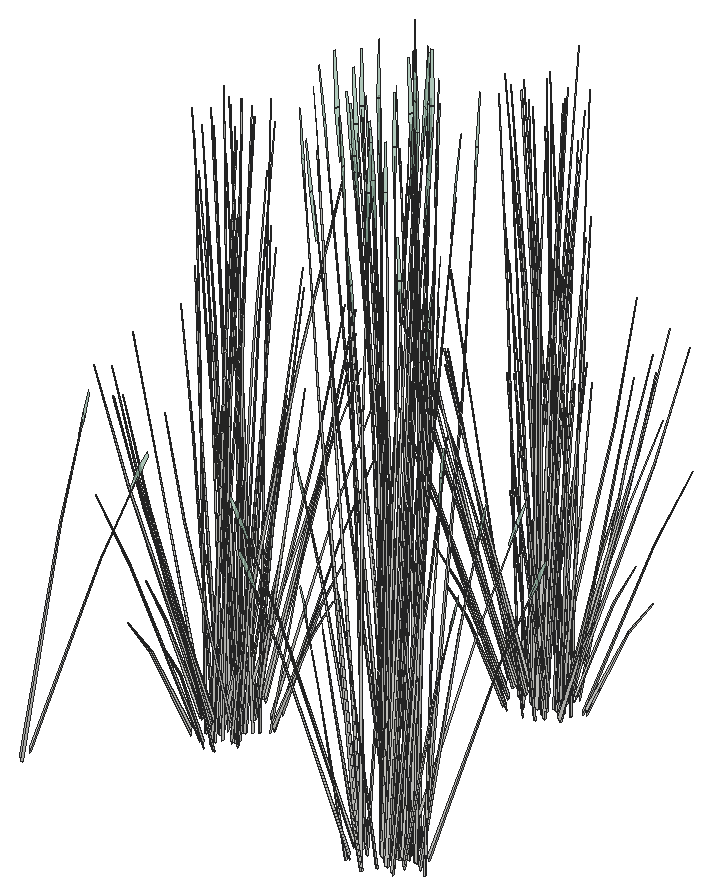
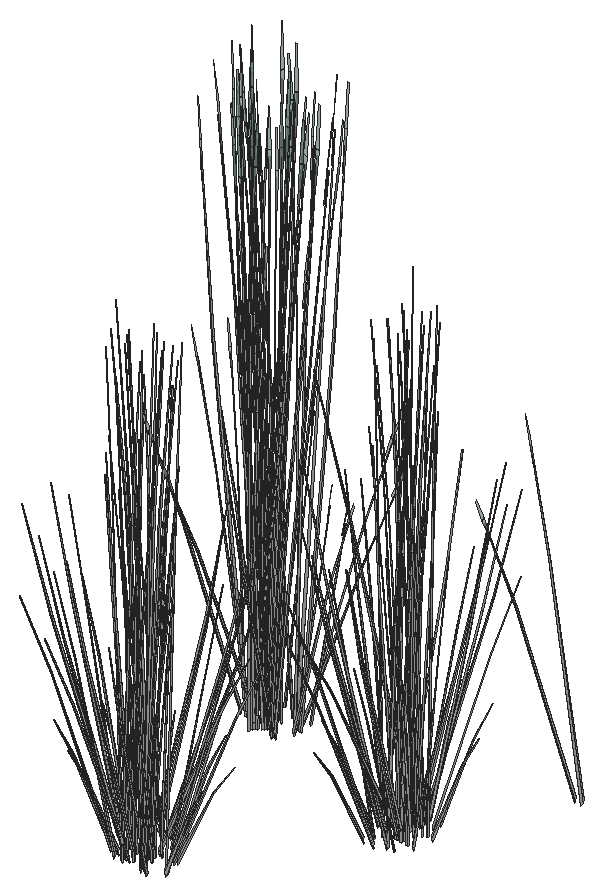
# SketchUp Ruby script. Lengths in inches.
U = 1.inch
M = Sketchup.active_model
def pt(a) = Geom::Point3d.new(a.map { |v| v * U })
def face(e, loops, mat)
  f = e.add_face(loops[0].map { |a| pt(a) })
  loops[1..].each { |l| e.add_face(l.map { |a| pt(a) }).erase! }
  f.material = f.back_material = mat if mat
  f
end
# faces: each face lists its corners as indices into pts; further lists are holes
def faces(e, pts, list, mat = nil) = list.each { |f| face(e, (f[0].is_a?(Array) ? f : [f]).map { |l| l.map { |i| pts[i] } }, mat) }
# xy, xz, yz: faces in a plane at the given z, y or x. An outline is a flat list of corners, or four numbers for a rectangle; further outlines are holes
def ring(l) = l.size == 4 ? [[l[0], l[1]], [l[2], l[1]], [l[2], l[3]], [l[0], l[3]]] : l.each_slice(2).to_a
def flat(e, list, mat, &to3) = list.each { |f| face(e, (f[0].is_a?(Array) ? f : [f]).map { |l| ring(l).map { |u, v| to3.(u, v) } }, mat) }
def xy(e, z, list, mat = nil) = flat(e, list, mat) { |x, y| [x, y, z] }
def xz(e, y, list, mat = nil) = flat(e, list, mat) { |x, z| [x, y, z] }
def yz(e, x, list, mat = nil) = flat(e, list, mat) { |y, z| [x, y, z] }
def lines(e, pts, list) = list.each { |a, b| e.add_line(pt(pts[a]), pt(pts[b])) }
# prism: a flat outline (further loops are holes) pulled along v
def prism(e, loops, v, mat = nil)
  f = face(e, loops, mat); d = Geom::Vector3d.new(v.map { |x| x * U })
  f.pushpull(f.normal.samedirection?(d) ? d.length : -d.length)
end
def box(e, o, s, mat = nil) = prism(e, [[o, [o[0] + s[0], o[1], o[2]], [o[0] + s[0], o[1] + s[1], o[2]], [o[0], o[1] + s[1], o[2]]]], [0, 0, s[2]], mat)
def at(x, y, z, deg = 0) = Geom::Transformation.translation(pt([x, y, z])) * Geom::Transformation.rotation(ORIGIN, Z_AXIS, deg.degrees)
def axes(o, x, y, z) = Geom::Transformation.new([*x, 0, *y, 0, *z, 0, *pt(o).to_a, 1])
def part(name) = M.definitions.add(name)
# library, detail: a bought-in or finely detailed component or shape, given as its bounding box
def library(name, o, s) = part(name).tap { |d| box(d.entities, o, s) }
def detail(e, o, s) = box(e.add_group.entities, o, s)
def put(e, d, t, mat = nil) = e.add_instance(d, t).tap { |i| i.material = mat if mat }
def group(e, t, mat = nil) = e.add_group.tap { |g| g.transformation = t; g.material = mat if mat }.entities
root = M.entities
M.materials.add("LightPink_Translucent").color = [175, 214, 192]
M.materials["LightPink_Translucent"].alpha = 0.75
c1 = part("blade")
p = [[2.15,0.21,22],[0,0.17,0],[0.09,0.45,0],[2.18,0.31,22],[2.29,0.31,22],[0.38,0.45,0],
  [2.48,0.24,33],[2.49,0.24,33],[2.48,0.22,33]]
faces(c1.entities,p,[[0,1,2,3],[4,5,2,3],[6,3,4,7],[8,0,3,6]])
c2 = part("seeds")
p = [[0.3,-0.1,1.38],[-0.01,-0.03,1.59],[-0.01,-0.03,0.03],[0.14,-0.07,-0.07],[0.29,-0.03,3],[0.15,0.01,3.11]]
faces(c2.entities,p,[[0,1,2,3],[1,0,4,5]],"LightPink_Translucent")
c3 = part("blade with seeds")
put(c3.entities,c1,at(0,0,0))
put(c3.entities,c2,axes([2.4,0.25,30.99],[1.5799,-0.05474,1.17369],[-0.12525,1.92788,0.29478],[-0.07173,-0.02425,1.56792]))
c4 = part("blade with seeds\#1")
put(c4.entities,c1,at(0,0,0))
put(root,c3,axes([465.83,231.75,139.07],[-0.30783,0.05344,1.28841],[-0.049,-0.4254,0.07375],[0.2156,-0.06439,0.73315]))
put(root,c3,axes([491.93,234.33,139.53],[-0.13585,0.09014,1.30132],[-0.40687,-0.15777,-0.27986],[0.07542,-0.19621,0.55638]))
put(root,c3,axes([489.83,234.16,139.53],[-0.02894,0.14568,1.30132],[-0.4231,0.12195,-0.27986],[-0.0989,-0.1883,0.55638]))
put(root,c3,axes([490.18,234.69,139.33],[-0.29882,-0.44625,0],[0.49993,-0.24886,-0.46963],[0.11386,-0.05668,1.48977]))
put(root,c3,axes([490.84,234.16,139.11],[-0.33028,0.25548,-0.03542],[-0.30262,-0.27981,-0.16061],[-0.02131,-0.07928,0.52975]))
put(root,c3,axes([465.92,232.38,139.62],[-0.1151,-0.10953,1.30132],[0.14976,-0.36232,-0.27986],[0.23288,0.04908,0.55638]))
put(root,c3,axes([493.24,235.39,139.53],[-0.17074,-0.01319,1.30132],[-0.17492,-0.35385,-0.27986],[0.20976,-0.1001,0.55638]))
put(root,c3,axes([489.2,234.62,139.11],[-0.13787,0.36364,-0.03542],[-0.42434,-0.11186,-0.16061],[-0.06443,-0.05948,0.52975]))
put(root,c3,axes([488.97,236.28,139.33],[-0.59763,0,0],[0,-0.49772,-0.46963],[0,-0.11336,1.48977]))
put(root,c3,axes([489.07,235.39,139.53],[0.09331,0.12399,1.30132],[-0.21502,0.33702,-0.27986],[-0.22079,-0.08055,0.55638]))
put(root,c3,axes([489.43,236.15,139.29],[-0.44456,0.37441,0.27988],[-0.44483,-0.37047,-0.33208],[-0.01552,-0.10632,1.50045]))
put(root,c3,axes([490.84,236.32,139.38],[0.53851,0.21584,0.21899],[-0.25917,0.44849,0.45502],[0,-0.10338,1.46094]))
put(root,c3,axes([490.63,236.93,139.39],[0.12668,-0.5277,-0.2132],[0.60063,0.09198,0.46656],[-0.10495,-0.07287,1.42361]))
put(root,c3,axes([489.33,236.36,139.43],[0,0.44533,0.45182],[-0.53472,0,0],[0,-0.10143,1.43328]))
put(root,c3,axes([492.38,234.81,139.33],[0.29882,-0.44625,0],[0.49993,0.24886,-0.46963],[0.11386,0.05668,1.48977]))
put(root,c3,axes([490.65,236.1875,139.32],[0.2078,0.49797,0.41637],[-0.59373,0.17316,0.16339],[0.00726,-0.0915,1.44559]))
put(root,c3,axes([493.56,236.57,138.97],[-0.30783,0.05344,1.28841],[-0.049,-0.4254,0.07375],[0.2156,-0.06439,0.73315]))
put(root,c3,axes([494.12,236.19,139.23],[-0.29631,-0.28477,-0.05904],[0.32453,-0.26092,-0.26768],[0.09195,-0.01837,0.88292]))
put(root,c3,axes([491.4,236.23,139.18],[0,-0.51528,0],[0.59763,0,0],[0,0,1.63305]))
put(root,c3,axes([492.125,235.04,139.43],[-0.44731,-0.22267,0.45182],[0.26736,-0.39927,0],[0.10188,0.05071,1.43328]))
put(root,c3,axes([491.12,235.91,139.32],[-0.39628,0.40415,0.41637],[-0.4708,-0.35675,0.16339],[0.09554,-0.04033,1.44559]))
put(root,c3,axes([491.55,236.63,139.26],[-0.44456,-0.3833,-0.05579],[0.44483,-0.38354,0],[-0.01552,-0.01339,1.5977]))
put(root,c3,axes([490.43,235.24,139.42],[-0.13807,0.44258,0.16054],[-0.50524,-0.12525,0.31929],[0.08728,-0.00216,1.4597]))
put(root,c3,axes([491.48,235.73,139.55],[0.0922,-0.39744,0.13176],[0.45047,0.06899,-0.37626],[0.08198,0.04081,1.15337]))
put(root,c3,axes([490.7,236.68,139.32],[0.60408,0.09383,0.41637],[-0.12294,0.52992,0.16339],[-0.08828,-0.05117,1.44559]))
put(root,c3,axes([490.38,237.52,139.42],[0.51358,-0.1182,0.16054],[0.12682,0.43988,0.31929],[-0.0458,-0.06409,1.4597]))
put(root,c3,axes([491.81,236.35,139.18],[0.53472,0,0],[0,0.46104,0],[0,0,1.6235]))
put(root,c3,axes([491.96,235.26,139.42],[-0.51358,0.1182,0.16054],[-0.12682,-0.43988,0.31929],[0.0458,0.06409,1.4597]))
put(root,c4,axes([474.01,240.52,138.84],[-0.09372,0.11973,1.17311],[-0.31002,-0.15578,-0.25229],[0.042,-0.24224,0.50157]))
put(root,c3,axes([491.63,236.11,139.34],[-0.60408,-0.09383,0.44771],[0.12294,-0.52992,0.17569],[0.08828,0.05117,1.5544]))
put(root,c3,axes([491.15,237.42,139.18],[-0.15594,-0.38394,0],[0.4453,-0.13445,0],[0,0,1.40478]))
put(root,c3,axes([490.85,237.06,139.55],[-0.0922,0.39744,0.13176],[-0.45047,-0.06899,-0.37626],[-0.08198,-0.04081,1.15337]))
put(root,c3,axes([491.73,237.37,139.16],[0.50177,-0.1511,-0.1747],[0.17632,0.43526,0.00007],[0.05539,-0.0167,1.58246]))
put(root,c3,axes([491.91,237.55,139.42],[0.13807,-0.44258,0.16054],[0.50524,0.12525,0.31929],[-0.08728,0.00216,1.4597]))
put(root,c3,axes([491.79,236.54,139.19],[0.33362,0.28765,0],[-0.33362,0.28765,0],[0,0,1.54032]))
put(root,c3,axes([492.7,236.42,139.42],[-0.37551,-0.32439,0.16054],[0.37842,-0.31463,0.31929],[-0.04147,0.06625,1.4597]))
put(root,c4,axes([473.5,241.19,140.8],[-0.16829,-0.43684,-0.58282],[0.34641,-0.24345,0.07033],[-0.03935,-0.21107,0.82446]))
put(root,c3,axes([491.04,237.59,139.17],[-0.48183,-0.19993,0],[0.23189,-0.41543,0],[0,0,1.48063]))
put(root,c3,axes([491.44,237.0625,139.41],[-0.4667,-0.35844,-0.22925],[0.39271,-0.40249,0.50168],[-0.12567,0.04193,1.53076]))
put(root,c3,axes([490.21,237.75,139.43],[0.44731,0.22267,0.45182],[-0.26736,0.39927,0],[-0.10188,-0.05071,1.43328]))
put(root,c3,axes([491.7,236.4375,139.26],[0,0.51503,-0.0513],[-0.59763,0,0],[0,0.01619,1.63225]))
put(root,c4,axes([474.2,241.62,140.8],[0.00917,-0.49695,-0.58282],[0.38634,0.03338,0.07033],[0.04077,-0.21053,0.82446]))
put(root,c3,axes([489.96,237.98,139.33],[-0.29882,0.44625,0],[-0.49993,-0.24886,-0.46963],[-0.11386,-0.05668,1.48977]))
put(root,c4,axes([473.6,239.95,138.99],[0.06291,0.30716,0.94226],[-0.25998,-0.14458,0.69231],[0.01779,-0.16295,0.20754]))
put(root,c4,axes([472.47,240.94,138.84],[-0.01129,0.1776,1.17311],[-0.30276,0.18194,-0.25229],[-0.08565,-0.21818,0.50157]))
put(root,c3,axes([493.01,236.43,139.43],[0,-0.44533,0.45182],[0.53472,0,0],[0,0.10143,1.43328]))
put(root,c3,axes([491.99,236.3,139.55],[0.4453,-0.12987,0.13176],[0.15594,0.37086,-0.37626],[0,0.08162,1.15337]))
put(root,c4,axes([473.375,241.11,140.56],[-0.34661,-0.13468,-0.41919],[0.1188,-0.46175,-0.3247],[-0.03178,-0.18591,0.80208]))
put(root,c3,axes([493.65,237.2,139.53],[-0.1151,-0.10953,1.30132],[0.14976,-0.36232,-0.27986],[0.23288,0.04908,0.55638]))
put(root,c3,axes([491.59,237.6,139.18],[0.48183,0.19993,0],[-0.23189,0.41543,0],[0,0,1.59208]))
put(root,c3,axes([491.78,238.04,139.17],[-0.29509,-0.44781,-0.04679],[0.49993,-0.24886,0.46963],[-0.12319,0.04264,1.48904]))
put(root,c3,axes([491.68,236.96,139.55],[0.3531,0.26757,0.13176],[-0.29453,0.30187,-0.37626],[-0.08198,0.04081,1.15337]))
put(root,c4,axes([472.74,241.32,140.8],[-0.30066,-0.25968,-0.58282],[0.21367,-0.45504,0.07033],[-0.10893,-0.15505,0.82446]))
put(root,c3,axes([492.05,237.78,139.43],[0.44731,-0.22267,0.45182],[0.26736,0.39927,0],[-0.10188,0.05071,1.43328]))
put(root,c3,axes([491.41,237.43,139.25],[0.2078,0.51161,-0.05471],[-0.59373,0.17927,0],[0.00726,0.01787,1.56677]))
put(root,c3,axes([488.43,237.2,139.53],[0.1661,0.03656,1.30132],[0.10705,0.37341,-0.27986],[-0.22562,0.0699,0.55638]))
put(root,c3,axes([493.37,236.51,139.33],[0.59763,0,0],[0,0.49772,-0.46963],[0,0.11336,1.48977]))
put(root,c3,axes([493.13,236.76,139.17],[-0.59734,-0.00356,-0.04529],[0,-0.49772,0.45448],[-0.01877,0.1133,1.441]))
put(root,c4,axes([471.91,240.74,138.99],[0.19397,0.16559,0.94226],[-0.26061,0.14233,0.69231],[-0.0653,-0.13676,0.20754]))
put(root,c4,axes([472.6,241.33,140.56],[-0.34793,0.12771,-0.41919],[-0.06086,-0.48364,-0.3247],[-0.09345,-0.1386,0.80208]))
put(root,c3,axes([491.79,237.8125,139.29],[0.59835,0.14475,0.27988],[-0.14969,0.51739,-0.33208],[-0.09903,0.06475,1.50045]))
put(root,c4,axes([474.65,242.29,140.56],[-0.09058,-0.49056,-0.41919],[0.34303,-0.08581,-0.3247],[0.0983,-0.13176,0.80208]))
put(root,c3,axes([492.16,238.09,139.33],[0.29882,0.44625,0],[-0.49993,0.24886,-0.46963],[-0.11386,0.05668,1.48977]))
put(root,c4,axes([475,241.61,138.91],[-0.01195,0.31879,0.86186],[-0.25381,-0.21053,0.47585],[0.09017,-0.12594,0.67605]))
put(root,c4,axes([474.5,241.65,138.99],[-0.10956,0.27991,0.94226],[-0.11132,-0.36143,0.69231],[0.0943,-0.09749,0.20754]))
put(root,c4,axes([474.38,242.65,138.84],[-0.12631,-0.00877,1.17311],[-0.14109,-0.41923,-0.25229],[0.15118,-0.12942,0.50157]))
put(root,c3,axes([491.6,237.63,139.53],[0.00843,-0.14762,1.30132],[0.40305,-0.1649,-0.27986],[0.12442,0.17669,0.55638]))
put(root,c4,axes([472.16,242.1,138.75],[-0.19052,0.46527,0.40731],[-0.34163,-0.2781,0],[0.04339,-0.10597,1.29208]))
put(root,c4,axes([473.35,241.1875,138.75],[-0.38104,0,0.40731],[0,-0.5562,0],[0.08679,0,1.29208]))
put(root,c4,axes([472.76,242.77,138.86],[-0.34006,-0.0959,0.11878],[0.05903,-0.46856,-0.33919],[0.03492,-0.08527,1.03975]))
put(root,c3,axes([489.52,238.29,139.74],[0.43418,-0.07886,0.05922],[0.09982,0.31771,-0.78537],[-0.02753,0.16083,0.70398]))
put(root,c4,axes([472.01,242.07,140.56],[-0.25603,0.35588,-0.41919],[-0.22422,-0.37594,-0.3247],[-0.13008,-0.05415,0.80208]))
put(root,c4,axes([472.85,242.97,138.95],[-0.31983,0.29864,0.36702],[-0.22522,-0.45236,-0.17663],[0.03957,-0.09664,1.17838]))
put(root,c4,axes([473.24,242.24,138.86],[-0.11112,-0.46318,0.11878],[0.31732,-0.1622,-0.33919],[0.06984,0,1.03975]))
put(root,c4,axes([473.08,242.61,138.67],[-0.08028,0.62833,0.4036],[-0.45342,-0.12787,0.15838],[0.04378,-0.09182,1.40127]))
put(root,c3,axes([489.41,238.63,139.53],[0.15082,-0.07025,1.30132],[0.37238,0.21183,-0.27986],[-0.11083,0.18329,0.55638]))
put(root,c4,axes([473.16,242.45,138.95],[-0.34335,-0.2412,0.36702],[0.16524,-0.50118,-0.17663],[0.07915,0,1.17838]))
put(root,c4,axes([474.81,243.375,140.56],[0.09552,-0.48869,-0.41919],[0.3275,0.16751,-0.3247],[0.13186,-0.04481,0.80208]))
put(root,c4,axes([472.9,243.15,138.65],[0.3458,0.41219,0.37535],[-0.30525,0.4897,0.14729],[-0.03451,-0.09937,1.30318]))
put(root,c4,axes([472.36,242.28,138.75],[0.10113,0.5342,0.14473],[-0.37638,0.13191,0.28783],[0.05484,-0.04764,1.3159]))
put(root,c4,axes([470.94,242.82,138.99],[0.2222,-0.06377,0.94226],[-0.12306,0.35378,0.69231],[-0.11377,-0.03807,0.20754]))
put(root,c4,axes([474.75,243.55,140.8],[0.30983,-0.23727,-0.58282],[0.17267,0.48842,0.07033],[0.1497,-0.05548,0.82446]))
put(root,c4,axes([473.34,241.51,138.75],[-0.27756,0.39059,0.14473],[-0.26921,-0.39362,0.28783],[0.05668,0.04314,1.3159]))
put(root,c4,axes([473.01,243.62,138.95],[0.02352,0.53984,0.36702],[-0.39046,0.04882,-0.17663],[-0.03957,-0.09664,1.17838]))
put(root,c4,axes([472.33,243.87,138.75],[0.37869,0.14361,0.14473],[-0.10717,0.52552,0.28783],[-0.00184,-0.09078,1.3159]))
put(root,c4,axes([473.26,243.43,138.71],[0.18468,-0.56014,0.19741],[0.38374,0.26958,0.41019],[-0.08846,0,1.31701]))
put(root,c4,axes([474.51,242.18,138.75],[-0.19052,-0.46527,0.40731],[0.34163,-0.2781,0],[0.04339,0.10597,1.29208]))
put(root,c4,axes([473.15,243.63,138.65],[0.42608,-0.21614,0.37535],[0.14817,0.61757,0.14729],[-0.07829,-0.00755,1.30318]))
put(root,c4,axes([474.31,242.33,138.75],[-0.37869,-0.14361,0.14473],[0.10717,-0.52552,0.28783],[0.00184,0.09078,1.3159]))
put(root,c4,axes([473.64,242.58,138.95],[-0.02352,-0.53984,0.36702],[0.39046,-0.04882,-0.17663],[0.03957,0.09664,1.17838]))
put(root,c4,axes([473.81,242.57,138.86],[0.22894,-0.36728,0.11878],[0.25829,0.30636,-0.33919],[0.03492,0.08527,1.03975]))
put(root,c4,axes([474.29,243.92,138.75],[-0.10113,-0.5342,0.14473],[0.37638,-0.13191,0.28783],[-0.05484,0.04764,1.3159]))
put(root,c4,axes([473.48,243.74,138.95],[0.34335,0.2412,0.36702],[-0.16524,0.50118,-0.17663],[-0.07915,0,1.17838]))
put(root,c4,axes([473.5625,243.58,138.65],[0.08028,-0.62833,0.37535],[0.45342,0.12787,0.14729],[-0.04378,0.09182,1.30318]))
put(root,c4,axes([471.76,243.125,140.56],[-0.09552,0.48869,-0.41919],[-0.3275,-0.16751,-0.3247],[-0.13186,0.04481,0.80208]))
put(root,c4,axes([473.26,242.34,139.05],[-0.35877,0.01358,1.15892],[0.093,-0.61462,0.4907],[0.19631,0.14537,1.09393]))
put(root,c4,axes([474.94,244.82,139.03],[-0.06748,-0.45162,0.05338],[0.27185,-0.10383,-0.708],[0.13761,0.02863,0.63462]))
put(root,c4,axes([473.89,243.43,138.86],[0.34006,0.0959,0.11878],[-0.05903,0.46856,-0.33919],[-0.03492,0.08527,1.03975]))
put(root,c4,axes([473.29,245.01,138.75],[0.38104,0,0.40731],[0,0.5562,0],[-0.08679,0,1.29208]))
put(root,c4,axes([474.48,244.09,138.75],[0.19052,-0.46527,0.40731],[0.34163,0.2781,0],[-0.04339,0.10597,1.29208]))
put(root,c4,axes([475.43,244.55,138.99],[-0.22657,0.01287,0.94226],[0.1616,-0.32149,0.69231],[0.10799,0.06323,0.20754]))
put(root,c4,axes([474.44,244.54,141.1],[0.35246,0.01294,-0.64693],[-0.02367,0.54471,0.07807],[0.14932,0.05748,0.91515]))
put(root,c4,axes([471.21,244.64,138.99],[0.13262,-0.25932,0.94226],[0.07972,0.37767,0.69231],[-0.10192,0.08081,0.20754]))
put(root,c4,axes([475.23,244.93,138.84],[-0.06011,-0.15688,1.17311],[0.18125,-0.38733,-0.25229],[0.15683,0.11528,0.50157]))
put(root,c4,axes([471.92,244.02,140.8],[-0.18418,0.4239,-0.58282],[-0.32274,-0.30126,0.07033],[-0.10997,0.15358,0.82446]))
put(root,c4,axes([471.92,244.21,140.56],[0.09058,0.49056,-0.41919],[-0.34303,0.08581,-0.3247],[-0.0983,0.13176,0.80208]))
put(root,c4,axes([473.97,245.17,140.56],[0.34793,-0.12771,-0.41919],[0.06086,0.48364,-0.3247],[0.09345,0.1386,0.80208]))
put(root,c4,axes([472.78,245.86,138.99],[-0.02727,-0.31739,0.94226],[0.24024,0.20133,0.69231],[-0.03604,0.15684,0.20754]))
put(root,c4,axes([474.68,246.31,138.99],[-0.1727,-0.20718,0.94226],[0.27339,-0.08175,0.69231],[0.04895,0.14972,0.20754]))
put(root,c4,axes([472.45,245.05,140.56],[0.25241,0.36098,-0.41919],[-0.26664,0.31614,-0.3247],[-0.0384,0.18341,0.80208]))
put(root,c4,axes([473.2,245.4,140.56],[0.34661,0.13468,-0.41919],[-0.1188,0.46175,-0.3247],[0.03178,0.18591,0.80208]))
put(root,c4,axes([472.37,244.88,140.8],[-0.00917,0.49695,-0.58282],[-0.38634,-0.03338,0.07033],[-0.04077,0.21053,0.82446]))
put(root,c4,axes([472.46,245.28,138.84],[0.10609,-0.09706,1.17311],[0.28837,0.22366,-0.25229],[-0.06892,0.22965,0.50157]))
put(root,c4,axes([472.99,244.42,139.46],[-0.05512,-0.14131,1.45254],[0.38487,-0.04873,0.11368],[0.05107,0.30608,0.51915]))
put(root,c4,axes([474.01,245.95,138.84],[0.03128,-0.17277,1.17311],[0.3195,-0.11135,-0.25229],[0.05981,0.23468,0.50157]))
put(root,c4,axes([487.07,256.04,138.84],[-0.14131,0.07713,1.17311],[-0.4232,-0.13499,-0.25229],[0.07845,-0.16789,0.50157]))
put(root,c4,axes([486.43,256.31,140.8],[-0.23727,-0.30983,-0.58282],[0.48842,-0.17267,0.07033],[-0.05548,-0.1497,0.82446]))
put(root,c4,axes([484.89,255.89,138.84],[-0.0301,0.12465,1.17311],[-0.44009,0.10435,-0.25229],[-0.10287,-0.16111,0.50157]))
put(root,c4,axes([487.42,256.61,140.8],[0.01294,-0.35246,-0.58282],[0.54471,0.02367,0.07033],[0.05748,-0.14932,0.82446]))
put(root,c4,axes([486.55,255.42,138.99],[0.06377,0.2222,0.94226],[-0.35378,-0.12306,0.69231],[0.03807,-0.11377,0.20754]))
put(root,c4,axes([486.25,256.24,140.56],[-0.48869,-0.09552,-0.41919],[0.16751,-0.3275,-0.3247],[-0.04481,-0.13186,0.80208]))
put(root,c4,axes([487.31,256.49,140.56],[-0.35588,-0.25603,-0.41919],[0.37594,-0.22422,-0.3247],[0.05415,-0.13008,0.80208]))
put(root,c4,axes([484.73,255.69,138.99],[0.25932,0.13262,0.94226],[-0.37767,0.07972,0.69231],[-0.08081,-0.10192,0.20754]))
put(root,c4,axes([485.36,256.39,140.8],[-0.4239,-0.18418,-0.58282],[0.30126,-0.32274,0.07033],[-0.15358,-0.10997,0.82446]))
put(root,c4,axes([485.16,256.4,140.56],[-0.49056,0.09058,-0.41919],[-0.08581,-0.34303,-0.3247],[-0.13176,-0.0983,0.80208]))
put(root,c4,axes([488.05,257.08,140.56],[-0.12771,-0.34793,-0.41919],[0.48364,-0.06086,-0.3247],[0.1386,-0.09345,0.80208]))
put(root,c4,axes([488.06,257.22,140.8],[0.25968,-0.30066,-0.58282],[0.45504,0.21367,0.07033],[0.15505,-0.10893,0.82446]))
put(root,c4,axes([488.43,256.95,138.84],[-0.1776,-0.01129,1.17311],[-0.18194,-0.30276,-0.25229],[0.21818,-0.08565,0.50157]))
put(root,c4,axes([488.64,256.39,138.99],[-0.16559,0.19397,0.94226],[-0.14233,-0.26061,0.69231],[0.13676,-0.0653,0.20754]))
put(root,c4,axes([484.09,256.94,138.84],[0.09706,0.10609,1.17311],[-0.22366,0.28837,-0.25229],[-0.22965,-0.06892,0.50157]))
put(root,c4,axes([484.5,256.85,140.8],[-0.49695,-0.00917,-0.58282],[0.03338,-0.38634,0.07033],[-0.21053,-0.04077,0.82446]))
put(root,c4,axes([484.33,256.93,140.56],[-0.36098,0.25241,-0.41919],[-0.31614,-0.26664,-0.3247],[-0.18341,-0.0384,0.80208]))
put(root,c4,axes([485.94,257.74,138.71],[0.56014,0.18468,0.19741],[-0.26958,0.38374,0.41019],[0,-0.08846,1.31701]))
put(root,c4,axes([483.52,257.26,138.99],[0.31739,-0.02727,0.94226],[-0.20133,0.24024,0.69231],[-0.15684,-0.03604,0.20754]))
put(root,c4,axes([485.76,257.48,138.95],[-0.53984,0.02352,0.36702],[-0.04882,-0.39046,-0.17663],[0.09664,-0.03957,1.17838]))
put(root,c4,axes([484.37,257.77,138.75],[0,0.38104,0.40731],[-0.5562,0,0],[0,-0.08679,1.29208]))
put(root,c4,axes([485.74,257.625,138.65],[0.21614,0.42608,0.37535],[-0.61757,0.14817,0.14729],[0.00755,-0.07829,1.30318]))
put(root,c4,axes([488.27,257.85,140.56],[0.13468,-0.34661,-0.41919],[0.46175,0.1188,-0.3247],[0.18591,-0.03178,0.80208]))
put(root,c4,axes([487.27,256.64,138.75],[-0.46527,-0.19052,0.40731],[0.2781,-0.34163,0],[0.10597,0.04339,1.29208]))
put(root,c4,axes([485.63,257.96,138.95],[-0.2412,0.34335,0.36702],[-0.50118,-0.16524,-0.17663],[0,-0.07915,1.17838]))
put(root,c4,axes([486.22,257.38,138.65],[-0.41219,0.3458,0.37535],[-0.4897,-0.30525,0.14729],[0.09937,-0.03451,1.30318]))
put(root,c4,axes([485.51,256.8125,138.75],[-0.14361,0.37869,0.14473],[-0.52552,-0.10717,0.28783],[0.09078,-0.00184,1.3159]))
put(root,c4,axes([488.18,257.98,140.8],[0.43684,-0.16829,-0.58282],[0.24345,0.34641,0.07033],[0.21107,-0.03935,0.82446]))
put(root,c4,axes([486.61,257.23,138.86],[0.0959,-0.34006,0.11878],[0.46856,0.05903,-0.33919],[0.08527,0.03492,1.03975]))
put(root,c4,axes([486.41,257.32,138.95],[-0.29864,-0.31983,0.36702],[0.45236,-0.22522,-0.17663],[0.09664,0.03957,1.17838]))
put(root,c4,axes([485.8,258.04,138.65],[0.62833,0.08028,0.37535],[-0.12787,0.45342,0.14729],[-0.09182,-0.04378,1.30318]))
put(root,c4,axes([487.1,256.83,138.75],[-0.5342,0.10113,0.14473],[-0.13191,-0.37638,0.28783],[0.04764,0.05484,1.3159]))
put(root,c4,axes([485.46,258.77,138.75],[0.5342,-0.10113,0.14473],[0.13191,0.37638,0.28783],[-0.04764,-0.05484,1.3159]))
put(root,c4,axes([486.76,257.56,138.67],[-0.62833,-0.08028,0.4036],[0.12787,-0.45342,0.15838],[0.09182,0.04378,1.40127]))
put(root,c4,axes([485.95,258.37,138.86],[-0.0959,0.34006,0.11878],[-0.46856,-0.05903,-0.33919],[-0.08527,-0.03492,1.03975]))
put(root,c4,axes([487.87,257.82,138.75],[-0.39059,-0.27756,0.14473],[0.39362,-0.26921,0.28783],[-0.04314,0.05668,1.3159]))
put(root,c4,axes([484.96,257.47,139.46],[0.14131,-0.05512,1.45254],[0.04873,0.38487,0.11368],[-0.30608,0.05107,0.51915]))
put(root,c4,axes([489.43,258.08,138.99],[-0.30716,0.06291,0.94226],[0.14458,-0.25998,0.69231],[0.16295,0.01779,0.20754]))
put(root,c4,axes([487.05,258.79,138.75],[0.14361,-0.37869,0.14473],[0.52552,0.10717,0.28783],[-0.09078,0.00184,1.3159]))
put(root,c4,axes([486.92,257.64,138.95],[0.2412,-0.34335,0.36702],[0.50118,0.16524,-0.17663],[0,0.07915,1.17838]))
put(root,c4,axes([485.28,258.96,138.75],[0.46527,0.19052,0.40731],[-0.2781,0.34163,0],[-0.10597,-0.04339,1.29208]))
put(root,c4,axes([483.98,257.68,140.56],[-0.13468,0.34661,-0.41919],[-0.46175,-0.1188,-0.3247],[-0.18591,0.03178,0.80208]))
put(root,c4,axes([488.1875,257.83,138.75],[0,-0.38104,0.40731],[0.5562,0,0],[0,0.08679,1.29208]))
put(root,c4,axes([487.13,257.72,138.86],[0.46318,-0.11112,0.11878],[0.1622,0.31732,-0.33919],[0,0.06984,1.03975]))
put(root,c4,axes([486.8,258.12,138.95],[0.53984,-0.02352,0.36702],[0.04882,0.39046,-0.17663],[-0.09664,0.03957,1.17838]))
put(root,c4,axes([488.85,258.49,138.84],[-0.11973,-0.09372,1.17311],[0.15578,-0.31002,-0.25229],[0.24224,0.042,0.50157]))
put(root,c4,axes([486.8,258.29,138.86],[0.36728,0.22894,0.11878],[-0.30636,0.25829,-0.33919],[-0.08527,0.03492,1.03975]))
put(root,c4,axes([487.76,258.68,140.8],[0.49695,0.00917,-0.58282],[-0.03338,0.38634,0.07033],[0.21053,0.04077,0.82446]))
put(root,c4,axes([487.2,258.99,138.75],[0.46527,-0.19052,0.40731],[0.2781,0.34163,0],[-0.10597,0.04339,1.29208]))
put(root,c4,axes([483.43,258.49,138.84],[0.17277,0.03128,1.17311],[0.11135,0.3195,-0.25229],[-0.23468,0.05981,0.50157]))
put(root,c4,axes([483.07,259.16,138.99],[0.20718,-0.1727,0.94226],[0.08175,0.27339,0.69231],[-0.14972,0.04895,0.20754]))
put(root,c4,axes([487.72,258.98,138.99],[-0.27991,-0.10956,0.94226],[0.36143,-0.11132,0.69231],[0.09749,0.0943,0.20754]))
put(root,c4,axes([484.21,258.45,140.56],[0.12771,0.34793,-0.41919],[-0.48364,0.06086,-0.3247],[-0.1386,0.09345,0.80208]))
put(root,c4,axes([487.04,257.74,139.05],[-0.01358,-0.35877,1.15892],[0.61462,0.093,0.4907],[-0.14537,0.19631,1.09393]))
put(root,c4,axes([487.09,259.13,140.56],[0.49056,-0.09058,-0.41919],[0.08581,0.34303,-0.3247],[0.13176,0.0983,0.80208]))
put(root,c4,axes([487.77,259.48,138.91],[-0.31879,-0.01195,0.86186],[0.21053,-0.25381,0.47585],[0.12594,0.09017,0.67605]))
put(root,c4,axes([486.73,258.86,138.84],[0.00877,-0.12631,1.17311],[0.41923,-0.14109,-0.25229],[0.12942,0.15118,0.50157]))
put(root,c4,axes([484.82,259.91,138.99],[-0.01287,-0.22657,0.94226],[0.32149,0.1616,0.69231],[-0.06323,0.10799,0.20754]))
put(root,c4,axes([486,259.29,140.56],[0.48869,0.09552,-0.41919],[-0.16751,0.3275,-0.3247],[0.04481,0.13186,0.80208]))
put(root,c4,axes([484.56,259.42,139.03],[0.45162,-0.06748,0.05338],[0.10383,0.27185,-0.708],[-0.02863,0.13761,0.63462]))
put(root,c4,axes([484.83,258.92,141.1],[-0.01294,0.35246,-0.64693],[-0.54471,-0.02367,0.07807],[-0.05748,0.14932,0.91515]))
